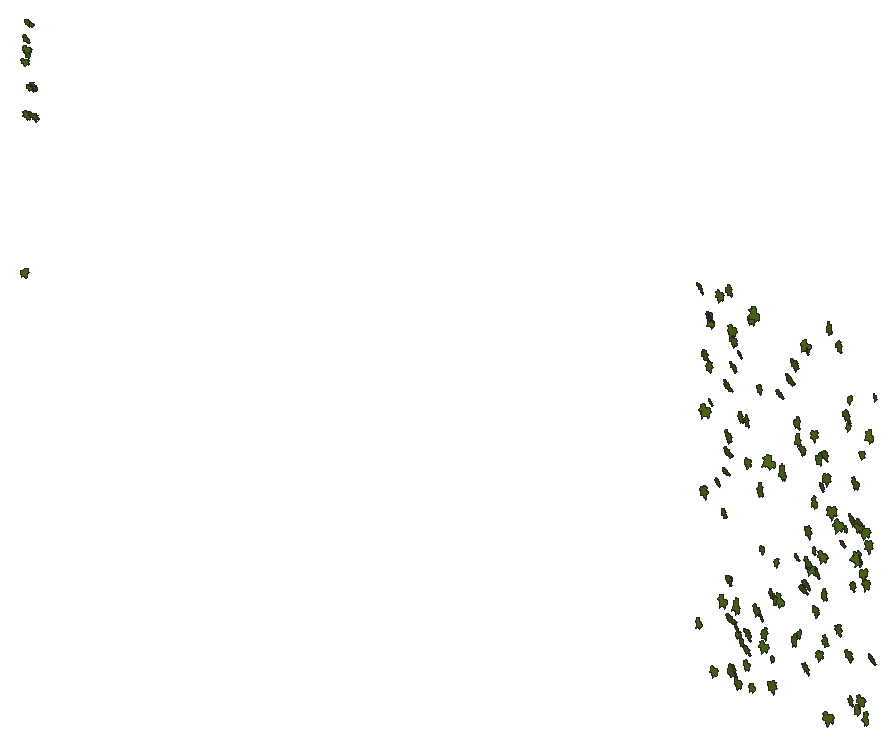
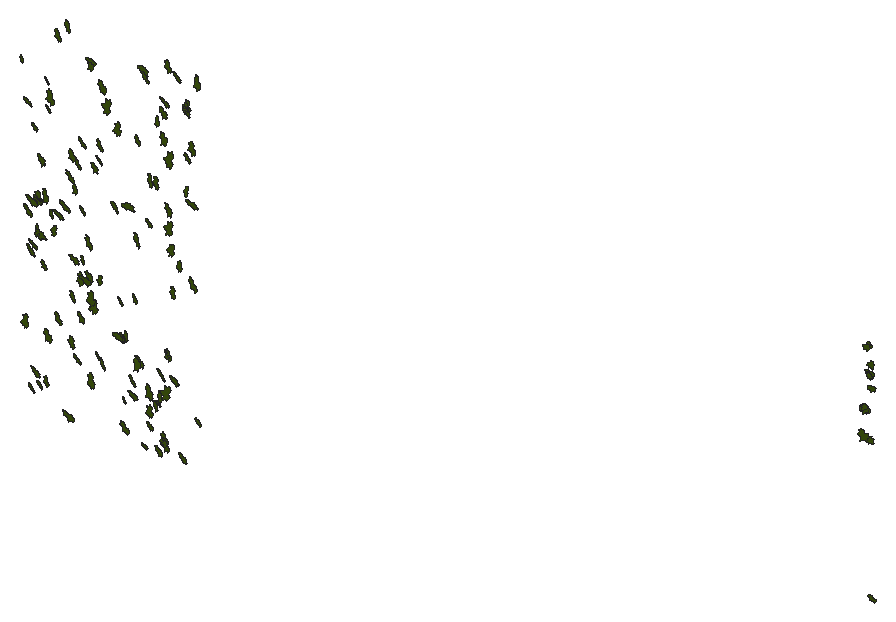
# SketchUp Ruby script. Lengths in inches.
U = 1.inch
M = Sketchup.active_model
def pt(a) = Geom::Point3d.new(a.map { |v| v * U })
def face(e, loops, mat)
  f = e.add_face(loops[0].map { |a| pt(a) })
  loops[1..].each { |l| e.add_face(l.map { |a| pt(a) }).erase! }
  f.material = f.back_material = mat if mat
  f
end
# faces: each face lists its corners as indices into pts; further lists are holes
def faces(e, pts, list, mat = nil) = list.each { |f| face(e, (f[0].is_a?(Array) ? f : [f]).map { |l| l.map { |i| pts[i] } }, mat) }
# xy, xz, yz: faces in a plane at the given z, y or x. An outline is a flat list of corners, or four numbers for a rectangle; further outlines are holes
def ring(l) = l.size == 4 ? [[l[0], l[1]], [l[2], l[1]], [l[2], l[3]], [l[0], l[3]]] : l.each_slice(2).to_a
def flat(e, list, mat, &to3) = list.each { |f| face(e, (f[0].is_a?(Array) ? f : [f]).map { |l| ring(l).map { |u, v| to3.(u, v) } }, mat) }
def xy(e, z, list, mat = nil) = flat(e, list, mat) { |x, y| [x, y, z] }
def xz(e, y, list, mat = nil) = flat(e, list, mat) { |x, z| [x, y, z] }
def yz(e, x, list, mat = nil) = flat(e, list, mat) { |y, z| [x, y, z] }
def lines(e, pts, list) = list.each { |a, b| e.add_line(pt(pts[a]), pt(pts[b])) }
# prism: a flat outline (further loops are holes) pulled along v
def prism(e, loops, v, mat = nil)
  f = face(e, loops, mat); d = Geom::Vector3d.new(v.map { |x| x * U })
  f.pushpull(f.normal.samedirection?(d) ? d.length : -d.length)
end
def box(e, o, s, mat = nil) = prism(e, [[o, [o[0] + s[0], o[1], o[2]], [o[0] + s[0], o[1] + s[1], o[2]], [o[0], o[1] + s[1], o[2]]]], [0, 0, s[2]], mat)
def at(x, y, z, deg = 0) = Geom::Transformation.translation(pt([x, y, z])) * Geom::Transformation.rotation(ORIGIN, Z_AXIS, deg.degrees)
def axes(o, x, y, z) = Geom::Transformation.new([*x, 0, *y, 0, *z, 0, *pt(o).to_a, 1])
def part(name) = M.definitions.add(name)
# library, detail: a bought-in or finely detailed component or shape, given as its bounding box
def library(name, o, s) = part(name).tap { |d| box(d.entities, o, s) }
def detail(e, o, s) = box(e.add_group.entities, o, s)
def put(e, d, t, mat = nil) = e.add_instance(d, t).tap { |i| i.material = mat if mat }
def group(e, t, mat = nil) = e.add_group.tap { |g| g.transformation = t; g.material = mat if mat }.entities
root = M.entities
M.materials.add("[Vegetation Blur 03]").color = [83, 114, 18]
c1 = part("ivy")
xy(c1.entities,0,[[0.782,0,0.786,0,0.787,0.005,0.789,0.009,0.821,0.072,0.875,0.147,1.001,0.272,1.073,0.331,1.137,0.363,1.178,0.379,1.223,0.384,1.272,0.383,1.311,0.374,1.36,0.355,1.399,0.334,1.491,0.285,1.541,0.244,1.583,0.199,1.617,0.15,1.64,0.128,1.662,0.115,1.717,0.105,1.745,0.093,1.784,0.054,1.819,0.057,1.854,0.064,1.882,0.075,1.896,0.074,1.91,0.071,1.937,0.063,1.964,0.053,1.99,0.038,2.016,0.015,2.034,0.002,2.04,0,2.038,0.003,2.036,0.007,2.033,0.038,2.036,0.068,2.045,0.1,2.055,0.116,2.064,0.123,2.077,0.129,2.088,0.129,2.106,0.132,2.118,0.13,2.179,0.132,2.207,0.133,2.225,0.133,2.242,0.138,2.22,0.162,2.207,0.186,2.206,0.213,2.212,0.236,2.228,0.262,2.247,0.274,2.298,0.283,2.355,0.294,2.37,0.296,2.376,0.295,2.377,0.3,2.377,0.303,2.385,0.329,2.411,0.37,2.426,0.392,2.449,0.407,2.511,0.426,2.561,0.444,2.619,0.466,2.589,0.469,2.561,0.476,2.501,0.5,2.449,0.516,2.424,0.523,2.401,0.535,2.377,0.556,2.372,0.568,2.36,0.575,2.268,0.586,2.225,0.592,2.207,0.599,2.194,0.61,2.143,0.65,2.13,0.664,2.122,0.682,2.123,0.7,2.13,0.719,2.148,0.75,2.17,0.781,2.195,0.807,2.221,0.828,2.284,0.874,2.291,0.88,2.288,0.887,2.276,0.9,2.267,0.916,2.265,0.933,2.273,0.967,2.292,1.002,2.313,1.03,2.334,1.054,2.348,1.067,2.358,1.074,2.363,1.076,2.362,1.081,2.35,1.094,2.347,1.11,2.35,1.143,2.359,1.18,2.385,1.254,2.415,1.324,2.448,1.393,2.45,1.4,2.446,1.398,2.44,1.394,2.427,1.383,2.402,1.36,2.376,1.339,2.345,1.324,2.305,1.309,2.282,1.303,2.273,1.306,2.245,1.294,2.212,1.287,2.187,1.291,2.163,1.301,2.142,1.316,2.134,1.327,2.124,1.325,2.09,1.292,2.053,1.259,2.014,1.234,1.973,1.215,1.954,1.21,1.931,1.208,1.909,1.212,1.893,1.22,1.879,1.233,1.872,1.248,1.867,1.281,1.864,1.319,1.821,1.258,1.773,1.197,1.726,1.141,1.698,1.121,1.679,1.116,1.666,1.117,1.647,1.122,1.632,1.129,1.62,1.141,1.617,1.154,1.617,1.219,1.621,1.254,1.623,1.268,1.623,1.281,1.618,1.314,1.606,1.346,1.603,1.375,1.607,1.403,1.603,1.467,1.599,1.499,1.605,1.525,1.614,1.552,1.629,1.577,1.635,1.589,1.629,1.587,1.618,1.582,1.596,1.566,1.581,1.556,1.568,1.552,1.557,1.55,1.545,1.553,1.531,1.562,1.522,1.572,1.504,1.591,1.486,1.611,1.474,1.631,1.457,1.666,1.455,1.684,1.457,1.698,1.452,1.715,1.444,1.728,1.424,1.754,1.419,1.772,1.423,1.786,1.434,1.819,1.444,1.848,1.446,1.855,1.44,1.861,1.43,1.867,1.386,1.904,1.349,1.948,1.326,1.973,1.31,1.995,1.288,2.048,1.284,2.153,1.287,2.254,1.284,2.255,1.282,2.253,1.278,2.247,1.274,2.237,1.266,2.216,1.226,2.125,1.208,2.076,1.184,2.033,1.155,1.984,1.135,1.942,1.111,1.899,1.083,1.861,1.053,1.85,1.059,1.83,1.061,1.809,1.056,1.79,1.049,1.767,1.04,1.749,1.018,1.733,0.994,1.726,0.942,1.734,0.95,1.6875,0.944,1.645,0.932,1.608,0.911,1.585,0.881,1.58,0.854,1.582,0.828,1.588,0.785,1.618,0.773,1.625,0.775,1.614,0.779,1.598,0.796,1.502,0.818,1.402,0.861,1.283,0.882,1.224,0.894,1.174,0.892,1.148,0.886,1.123,0.881,1.107,0.872,1.099,0.849,1.094,0.818,1.092,0.789,1.098,0.762,1.107,0.753,1.113,0.721,1.139,0.698,1.163,0.678,1.194,0.665,1.224,0.628,1.28,0.612,1.312,0.606,1.327,0.606,1.314,0.599,1.282,0.594,1.267,0.581,1.256,0.544,1.245,0.512,1.244,0.473,1.249,0.444,1.256,0.382,1.288,0.339,1.306,0.324,1.316,0.317,1.324,0.309,1.326,0.27,1.314,0.227,1.313,0.185,1.3125,0.152,1.317,0.122,1.328,0.092,1.345,0.073,1.353,0.079,1.338,0.092,1.308,0.117,1.249,0.13,1.215,0.139,1.164,0.147,1.148,0.157,1.136,0.163,1.122,0.174,1.086,0.177,1.067,0.182,1.054,0.186,1.043,0.191,1.038,0.211,1.028,0.237,1.005,0.25,0.974,0.253,0.96,0.25,0.944,0.242,0.914,0.243,0.906,0.249,0.902,0.26,0.894,0.289,0.88,0.307,0.873,0.322,0.862,0.364,0.799,0.403,0.738,0.431,0.709,0.439,0.691,0.441,0.678,0.4375,0.66,0.428,0.645,0.394,0.623,0.303,0.594,0.255,0.581,0.214,0.577,0.179,0.573,0.173,0.568,0.175,0.561,0.167,0.55,0.141,0.523,0.113,0.503,0.077,0.49,0.045,0.486,0.026,0.485,0.019,0.486,0.011,0.483,0,0.471,0.014,0.467,0.044,0.455,0.058,0.447,0.07,0.438,0.097,0.411,0.125,0.394,0.158,0.377,0.174,0.366,0.182,0.359,0.185,0.361,0.242,0.331,0.253,0.316,0.258,0.303,0.262,0.283,0.274,0.278,0.308,0.274,0.341,0.252,0.366,0.226,0.366,0.222,0.37,0.22,0.38,0.221,0.395,0.221,0.425,0.216,0.45,0.207,0.465,0.192,0.473,0.178,0.484,0.15,0.489,0.116,0.483,0.089,0.468,0.058,0.45,0.035,0.435,0.018,0.429,0.011,0.434,0.012,0.438,0.014,0.469,0.019,0.542,0.016,0.581,0.015,0.612,0.027,0.68,0.055,0.696,0.057,0.712,0.052,0.73,0.045,0.741,0.036,0.766,0.014]])
put(root,c1,axes([31.32,173.2,140.17],[0.36239,0.03439,0.0325],[0.04011,-0.01114,-0.29602],[0.01602,-0.75014,0.00588]),"[Vegetation Blur 03]")
put(root,c1,axes([31.76,173.2,143.07],[0.31224,-0.04153,-0.22289],[-0.2695,0.10455,-0.25454],[-0.04857,-0.84719,-0.02048]),"[Vegetation Blur 03]")
put(root,c1,axes([31.16,173.2,116.41],[0.30062,0.06409,0.25513],[0.31279,-0.14376,-0.23982],[-0.02918,-0.88082,0.05771]),"[Vegetation Blur 03]")
put(root,c1,axes([32.02,173.2,134.62],[0.2286,-0.00259,-0.27195],[-0.33307,0.02295,-0.18652],[-0.00991,-0.83122,-0.0043]),"[Vegetation Blur 03]")
put(root,c1,axes([32.45,173.2,141.72],[0.11758,-0.14394,-0.33997],[-0.41694,0.10295,-0.1029],[-0.06765,-0.88473,0.04334]),"[Vegetation Blur 03]")
put(root,c1,axes([31.58,173.2,141.8],[0.42779,-0.01722,0.00276],[0.0027,-0.07154,-0.34805],[-0.00862,-0.87743,0.02832]),"[Vegetation Blur 03]")
put(root,c1,axes([31.75,173.2,144.62],[0.24814,-0.07421,0.13501],[0.16554,-0.02052,-0.20443],[-0.03556,-0.61336,-0.0095]),"[Vegetation Blur 03]")
put(root,c1,axes([32.1,173.2,144.75],[0.32819,0.01887,-0.10221],[-0.12554,0.06541,-0.2666],[-0.0028,-0.71988,-0.0269]),"[Vegetation Blur 03]")
put(root,c1,axes([31.87,173.2,137.29],[0.29759,0.01634,0.29239],[0.3571,0.0663,-0.24267],[0.02985,-0.95609,-0.01183]),"[Vegetation Blur 03]")
put(root,c1,axes([32.18,173.2,137.7],[0.43208,-0.00485,-0.01137],[-0.01346,0.125,-0.34915],[-0.00429,-0.88078,-0.04949]),"[Vegetation Blur 03]")
put(root,c1,axes([32.07,173.2,134.58],[0.54527,-0.10858,0.11727],[0.14945,0.14116,-0.4423],[-0.03309,-1.15173,-0.06527]),"[Vegetation Blur 03]")
put(root,c1,axes([115.06,173.7,107.27],[0.44114,-0.2833,-0.10477],[-0.14493,-0.08165,-0.37173],[-0.12012,-0.94191,0.06374]),"[Vegetation Blur 03]")
put(root,c1,axes([114.86,173.7,144.42],[0.47356,-0.40672,0.26845],[0.33871,-0.06229,-0.41283],[-0.18036,-1.18486,-0.07045]),"[Vegetation Blur 03]")
put(root,c1,axes([115.53,173.7,131.28],[0.64635,-0.1795,-0.0483],[-0.07498,-0.25102,-0.52154],[-0.0741,-1.31182,0.10641]),"[Vegetation Blur 03]")
put(root,c1,axes([115.22,173.7,121.76],[0.52711,-0.21147,0.33505],[0.39283,-0.25745,-0.4372],[-0.15742,-1.35053,0.03088]),"[Vegetation Blur 03]")
put(root,c1,axes([115.43,173.7,136.7],[0.32628,-0.20206,0.40603],[0.49033,-0.18475,-0.27691],[-0.12932,-1.21026,-0.02552]),"[Vegetation Blur 03]")
put(root,c1,axes([116.1,173.7,141.6],[0.40522,-0.15446,0.13943],[0.15914,-0.15283,-0.3347],[-0.09744,-0.89194,0.0332]),"[Vegetation Blur 03]")
put(root,c1,axes([116.03,173.7,135.72],[0.34108,-0.07651,0.26436],[0.30846,-0.23678,-0.27587],[-0.10562,-0.93855,0.04805]),"[Vegetation Blur 03]")
put(root,c1,axes([116.6,173.7,141.49],[0.45619,-0.27219,-0.21417],[-0.27378,-0.03129,-0.38217],[-0.10679,-1.08253,0.0649]),"[Vegetation Blur 03]")
put(root,c1,axes([116.54,173.7,131.73],[0.12614,-0.2409,0.28031],[0.3435,-0.16191,-0.12485],[-0.11696,-0.73532,-0.06434]),"[Vegetation Blur 03]")
put(root,c1,axes([116.49,173.7,140.97],[0.11866,-0.26117,0.39663],[0.48542,-0.20436,-0.1179],[-0.12904,-1.00894,-0.07879]),"[Vegetation Blur 03]")
put(root,c1,axes([116.65,173.7,102.41],[0.52824,-0.2088,0.07813],[0.0803,-0.17577,-0.43551],[-0.11407,-1.09065,0.05523]),"[Vegetation Blur 03]")
put(root,c1,axes([117.2,173.7,123.2],[0.23432,-0.21265,0.28086],[0.3439,-0.11223,-0.20448],[-0.10411,-0.84934,-0.0433]),"[Vegetation Blur 03]")
put(root,c1,axes([117.39,173.7,144.48],[0.53111,-0.22481,0.11811],[0.12292,-0.23121,-0.43739],[-0.1333,-1.10892,0.06725]),"[Vegetation Blur 03]")
put(root,c1,axes([117.9,173.7,110.91],[0.58633,-0.27865,-0.1062],[-0.1477,-0.14213,-0.48453],[-0.11598,-1.22771,0.08019]),"[Vegetation Blur 03]")
put(root,c1,axes([117.98,173.7,119.81],[0.1731,-0.14266,0.38005],[0.45428,-0.21748,-0.15066],[-0.12362,-0.99891,-0.02148]),"[Vegetation Blur 03]")
put(root,c1,axes([118.19,173.7,124.49],[0.13916,-0.21976,0.37305],[0.46529,-0.06512,-0.12164],[-0.06205,-0.98109,-0.07549]),"[Vegetation Blur 03]")
put(root,c1,axes([118.49,173.7,126.62],[0.10022,-0.2222,0.4688],[0.57871,-0.13035,-0.09212],[-0.08191,-1.19279,-0.07727]),"[Vegetation Blur 03]")
put(root,c1,axes([118.39,173.7,129.41],[0.62179,-0.3866,0.07255],[0.08725,-0.03824,-0.53009],[-0.18864,-1.29198,-0.00602]),"[Vegetation Blur 03]")
put(root,c1,axes([118.45,173.7,112.9],[0.37075,-0.20222,0.27738],[0.33431,-0.13128,-0.31269],[-0.11578,-1.02663,-0.01465]),"[Vegetation Blur 03]")
put(root,c1,axes([118.4375,173.7,144.87],[0.27432,-0.11887,0.39101],[0.46845,-0.2067,-0.22879],[-0.11587,-1.1171,0.00072]),"[Vegetation Blur 03]")
put(root,c1,axes([118.4,173.7,134.14],[0.18149,-0.29755,0.51892],[0.63719,-0.20751,-0.16715],[-0.13848,-1.34475,-0.08903]),"[Vegetation Blur 03]")
put(root,c1,axes([118.8,173.7,112.98],[0.30081,-0.15518,0.1985],[0.21889,-0.23826,-0.25024],[-0.13012,-0.75955,0.03794]),"[Vegetation Blur 03]")
put(root,c1,axes([118.8125,173.7,108.14],[0.09309,-0.2572,0.47512],[0.59358,-0.05541,-0.08218],[-0.0469,-1.21192,-0.09707]),"[Vegetation Blur 03]")
put(root,c1,axes([118.6875,173.7,102.4],[0.19741,-0.09695,0.50499],[0.60705,-0.24693,-0.16553],[-0.12869,-1.3135,-0.00615]),"[Vegetation Blur 03]")
put(root,c1,axes([118.93,173.7,141.25],[0.5878,-0.24093,0.03931],[0.02588,-0.23212,-0.48155],[-0.12393,-1.19122,0.08588]),"[Vegetation Blur 03]")
put(root,c1,axes([118.9375,173.7,137.15],[0.5598,-0.34639,0.09978],[0.13771,0.07562,-0.47332],[-0.15594,-1.17668,-0.05979]),"[Vegetation Blur 03]")
put(root,c1,axes([119,173.7,140.08],[0.56579,-0.26175,0.06944],[0.08066,-0.05979,-0.47321],[-0.13005,-1.17586,0.0086]),"[Vegetation Blur 03]")
put(root,c1,axes([119.02,173.7,103.04],[0.3696,-0.27711,0.38105],[0.45779,-0.2062,-0.31935],[-0.16294,-1.2079,-0.0329]),"[Vegetation Blur 03]")
put(root,c1,axes([119.96,173.7,111.21],[0.5074,-0.4678,-0.2898],[-0.37384,0.02954,-0.44347],[-0.19497,-1.27408,0.09613]),"[Vegetation Blur 03]")
put(root,c1,axes([119.83,173.7,107.24],[0.27201,-0.08351,0.1346],[0.14493,-0.22002,-0.21655],[-0.08857,-0.61651,0.05905]),"[Vegetation Blur 03]")
put(root,c1,axes([119.73,173.7,107.69],[0.16819,-0.22664,0.32974],[0.39401,-0.21788,-0.15742],[-0.14187,-0.87383,-0.04627]),"[Vegetation Blur 03]")
put(root,c1,axes([119.64,173.7,102.19],[0.53858,-0.252,0.05397],[0.05479,-0.1161,-0.44944],[-0.12794,-1.11057,0.03474]),"[Vegetation Blur 03]")
put(root,c1,axes([119.98,173.7,138.58],[0.31604,-0.28517,0.16056],[0.20748,-0.01555,-0.27638],[-0.12189,-0.7659,-0.05417]),"[Vegetation Blur 03]")
put(root,c1,axes([120.3,173.7,107.26],[0.4884,-0.38994,-0.09349],[-0.11293,0.05241,-0.42733],[-0.19047,-1.03097,0.01363]),"[Vegetation Blur 03]")
put(root,c1,axes([120.05,173.7,131.25],[0.21062,-0.15839,0.41958],[0.49728,-0.27124,-0.18238],[-0.15148,-1.11064,-0.0153]),"[Vegetation Blur 03]")
put(root,c1,axes([120.87,173.7,104.6],[0.49081,-0.25055,0.00673],[-0.00728,-0.13032,-0.40947],[-0.12182,-1.0017,0.05159]),"[Vegetation Blur 03]")
put(root,c1,axes([120.72,173.7,105.65],[0.28606,-0.20547,0.36321],[0.44363,-0.1257,-0.24391],[-0.10592,-1.08138,-0.04066]),"[Vegetation Blur 03]")
put(root,c1,axes([120.91,173.7,127.01],[0.44605,-0.17185,0.11357],[0.12178,-0.19918,-0.36599],[-0.10728,-0.94065,0.05675]),"[Vegetation Blur 03]")
put(root,c1,axes([120.78,173.7,131.1875],[0.25712,-0.18798,0.42224],[0.4923,-0.32764,-0.22263],[-0.18343,-1.14283,-0.00563]),"[Vegetation Blur 03]")
put(root,c1,axes([120.73,173.7,107.98],[0.55958,-0.3731,0.26041],[0.3198,-0.09162,-0.47837],[-0.18004,-1.32239,-0.04033]),"[Vegetation Blur 03]")
put(root,c1,axes([121.6875,173.7,102.27],[0.36884,-0.18268,-0.08765],[-0.12074,-0.10682,-0.30338],[-0.06956,-0.78327,0.06182]),"[Vegetation Blur 03]")
put(root,c1,axes([121.17,173.7,142.66],[0.3032,0.00804,0.42723],[0.50376,-0.343,-0.23711],[-0.14236,-1.19666,0.07083]),"[Vegetation Blur 03]")
put(root,c1,axes([122.01,173.7,144.4],[0.54958,-0.28156,-0.28314],[-0.3622,-0.10008,-0.45262],[-0.08884,-1.33367,0.09374]),"[Vegetation Blur 03]")
put(root,c1,axes([121.97,173.7,111.18],[0.5531,-0.30937,0.07702],[0.082,-0.11827,-0.46698],[-0.15743,-1.14854,0.02734]),"[Vegetation Blur 03]")
put(root,c1,axes([122.3,173.7,135.49],[0.34266,-0.16677,0.2483],[0.29126,-0.18349,-0.28712],[-0.11956,-0.92493,0.01219]),"[Vegetation Blur 03]")
put(root,c1,axes([122.31,173.7,110.93],[0.62192,-0.51222,0.08279],[0.13225,0.12501,-0.54004],[-0.23401,-1.29066,-0.08517]),"[Vegetation Blur 03]")
put(root,c1,axes([122.38,173.7,123.84],[0.18528,-0.05644,0.53215],[0.61865,-0.42892,-0.15063],[-0.2078,-1.32731,0.02605]),"[Vegetation Blur 03]")
put(root,c1,axes([122.76,173.7,117.9],[0.3651,-0.20886,0.13721],[0.15459,-0.14475,-0.30864],[-0.12111,-0.81437,0.01967]),"[Vegetation Blur 03]")
put(root,c1,axes([122.87,173.7,107.41],[0.56213,-0.17838,-0.00831],[-0.02255,-0.16495,-0.45927],[-0.08432,-1.14512,0.06745]),"[Vegetation Blur 03]")
put(root,c1,axes([122.9,173.7,108.37],[0.33688,-0.08622,0.33874],[0.38873,-0.33347,-0.27086],[-0.15137,-1.04826,0.0583]),"[Vegetation Blur 03]")
put(root,c1,axes([123.91,173.7,128.56],[0.49181,-0.15671,-0.3315],[-0.41314,-0.21702,-0.39213],[0.00973,-1.29451,0.10587]),"[Vegetation Blur 03]")
put(root,c1,axes([123.92,173.7,112.97],[0.15407,-0.1087,0.33806],[0.39127,-0.27976,-0.13293],[-0.14585,-0.86534,0.00051]),"[Vegetation Blur 03]")
put(root,c1,axes([124.18,173.7,106.15],[0.27567,-0.18278,0.07916],[0.08,-0.13493,-0.23455],[-0.1044,-0.58604,0.02931]),"[Vegetation Blur 03]")
put(root,c1,axes([123.63,173.7,102.98],[0.51611,-0.14167,0.29822],[0.35265,-0.22138,-0.42305],[-0.1179,-1.28232,0.04009]),"[Vegetation Blur 03]")
put(root,c1,axes([124.38,173.7,113.2],[0.43914,-0.29657,0.03896],[0.03337,-0.10478,-0.37595],[-0.14811,-0.90294,0.03083]),"[Vegetation Blur 03]")
put(root,c1,axes([124.51,173.7,116.86],[0.29156,-0.09126,0.22735],[0.25627,-0.25873,-0.23525],[-0.11785,-0.78843,0.05088]),"[Vegetation Blur 03]")
put(root,c1,axes([125.12,173.7,113.54],[0.50163,-0.24569,-0.26541],[-0.34021,-0.12729,-0.40976],[-0.06534,-1.2236,0.09592]),"[Vegetation Blur 03]")
put(root,c1,axes([124.75,173.7,135.72],[0.30187,-0.29092,0.34167],[0.43037,-0.04293,-0.25902],[-0.10016,-1.06123,-0.08319]),"[Vegetation Blur 03]")
put(root,c1,axes([125.66,173.7,128.05],[0.48032,-0.40321,-0.3461],[-0.42858,0.11763,-0.41773],[-0.18586,-1.31325,0.06885]),"[Vegetation Blur 03]")
put(root,c1,axes([126.23,173.7,137.39],[0.07798,-0.22712,0.49701],[0.61066,-0.17712,-0.07655],[-0.10063,-1.25091,-0.0794]),"[Vegetation Blur 03]")
put(root,c1,axes([126.5,173.7,140.07],[0.58958,-0.29849,0.19052],[0.22934,-0.09222,-0.49546],[-0.15145,-1.30163,-0.00859]),"[Vegetation Blur 03]")
put(root,c1,axes([126.63,173.7,108.75],[0.26152,-0.04302,0.44662],[0.5117,-0.42542,-0.20602],[-0.19512,-1.17335,0.05832]),"[Vegetation Blur 03]")
put(root,c1,axes([127.14,173.7,118.17],[0.15681,-0.19135,0.27864],[0.34217,-0.11382,-0.14055],[-0.09017,-0.7647,-0.0488]),"[Vegetation Blur 03]")
put(root,c1,axes([126.93,173.7,133.11],[0.28904,-0.06987,0.39444],[0.46239,-0.30604,-0.23421],[-0.14468,-1.11768,0.03947]),"[Vegetation Blur 03]")
put(root,c1,axes([127.56,173.7,132.16],[0.42016,-0.3703,-0.17602],[-0.23818,-0.04638,-0.36333],[-0.14889,-0.97076,0.0845]),"[Vegetation Blur 03]")
put(root,c1,axes([127.36,173.7,109.79],[0.24227,-0.06001,0.24324],[0.27574,-0.26297,-0.19314],[-0.11679,-0.74533,0.04856]),"[Vegetation Blur 03]")
put(root,c1,axes([127.63,173.7,130.96],[0.51145,-0.25079,0.06105],[0.06998,-0.0596,-0.42899],[-0.12471,-1.06199,0.00966]),"[Vegetation Blur 03]")
put(root,c1,axes([127.61,173.7,114.92],[0.32867,-0.28906,0.36046],[0.45664,0.0115,-0.27589],[-0.07923,-1.13284,-0.09478]),"[Vegetation Blur 03]")
put(root,c1,axes([128.24,173.7,142.85],[0.51677,-0.16,-0.11108],[-0.14975,-0.2188,-0.41446],[-0.04632,-1.0777,0.10064]),"[Vegetation Blur 03]")
put(root,c1,axes([128.12,173.7,142.01],[0.40968,-0.27629,0.16507],[0.21084,0.00024,-0.34848],[-0.12034,-0.94019,-0.0486]),"[Vegetation Blur 03]")
put(root,c1,axes([127.94,173.7,115.6875],[0.38346,-0.30784,0.36497],[0.45646,-0.05536,-0.32679],[-0.11835,-1.21097,-0.07784]),"[Vegetation Blur 03]")
put(root,c1,axes([128.41,173.7,118.82],[0.56324,-0.31646,-0.09717],[-0.11977,0.02711,-0.47626],[-0.15324,-1.18433,0.01506]),"[Vegetation Blur 03]")
put(root,c1,axes([127.96,173.7,106.5],[0.44878,-0.3413,0.36007],[0.4395,-0.14984,-0.38721],[-0.17027,-1.28634,-0.05043]),"[Vegetation Blur 03]")
put(root,c1,axes([128.26,173.7,121.87],[0.47957,-0.26061,0.31785],[0.37221,-0.23733,-0.40467],[-0.1708,-1.24893,0.01057]),"[Vegetation Blur 03]")
put(root,c1,axes([128.76,173.7,118.26],[0.59751,-0.1415,-0.08723],[-0.11552,-0.16395,-0.48523],[-0.05298,-1.23827,0.07421]),"[Vegetation Blur 03]")
put(root,c1,axes([129.55,173.7,125.92],[0.4464,-0.35085,-0.18371],[-0.23796,-0.0009,-0.38487],[-0.15203,-1.02878,0.06299]),"[Vegetation Blur 03]")
put(root,c1,axes([129.26,173.7,119.75],[0.21308,-0.12887,0.25392],[0.29486,-0.2048,-0.18116],[-0.11737,-0.74847,0.00585]),"[Vegetation Blur 03]")
put(root,c1,axes([129.1,173.7,132.9],[0.46976,-0.15316,0.21327],[0.23871,-0.28032,-0.3819],[-0.12977,-1.07007,0.06952]),"[Vegetation Blur 03]")
put(root,c1,axes([129.29,173.7,113.51],[0.49387,-0.24848,0.14861],[0.17062,-0.13992,-0.41447],[-0.13648,-1.07408,0.01961]),"[Vegetation Blur 03]")
put(root,c1,axes([129.4,173.7,117.45],[0.34584,-0.27967,0.31588],[0.38688,-0.124,-0.2994],[-0.13639,-1.06088,-0.04828]),"[Vegetation Blur 03]")
put(root,c1,axes([129.66,173.7,130.13],[0.31073,-0.06738,0.37222],[0.4328,-0.32267,-0.24985],[-0.14749,-1.08882,0.05101]),"[Vegetation Blur 03]")
put(root,c1,axes([129.79,173.7,108.68],[0.45593,-0.14871,0.15697],[0.17169,-0.25336,-0.36992],[-0.11285,-0.98625,0.07136]),"[Vegetation Blur 03]")
put(root,c1,axes([130.1,173.7,127.4375],[0.37901,-0.24998,0.16924],[0.20826,-0.05609,-0.32368],[-0.11995,-0.88726,-0.02722]),"[Vegetation Blur 03]")
put(root,c1,axes([130.1,173.7,119.98],[0.58607,-0.17658,0.01299],[0.00501,-0.15402,-0.47969],[-0.08713,-1.19658,0.05983]),"[Vegetation Blur 03]")
put(root,c1,axes([130.4,173.7,114.98],[0.16191,-0.03187,0.41572],[0.48687,-0.31523,-0.1301],[-0.15054,-1.05373,0.02635]),"[Vegetation Blur 03]")
put(root,c1,axes([130.36,173.7,130.95],[0.39018,-0.19806,0.28181],[0.33951,-0.13277,-0.32778],[-0.115,-1.06391,-0.01155]),"[Vegetation Blur 03]")
put(root,c1,axes([130.5,173.7,109.8125],[0.12637,-0.06641,0.44261],[0.52763,-0.25805,-0.10643],[-0.12947,-1.11645,-0.00173]),"[Vegetation Blur 03]")
put(root,c1,axes([130.51,173.7,128.55],[0.51632,-0.17161,0.26126],[0.29868,-0.283,-0.42241],[-0.14219,-1.21766,0.06135]),"[Vegetation Blur 03]")
put(root,c1,axes([130.65,173.7,102.21],[0.65317,-0.15035,0.08957],[0.09783,-0.2124,-0.5313],[-0.08838,-1.34629,0.07382]),"[Vegetation Blur 03]")
put(root,c1,axes([131.04,173.7,144.75],[0.0835,-0.00667,0.46395],[0.54474,-0.33722,-0.06606],[-0.16259,-1.13325,0.01693]),"[Vegetation Blur 03]")
put(root,c1,axes([131.07,173.7,125.15],[0.58365,-0.1286,0.23072],[0.26562,-0.28309,-0.47237],[-0.11521,-1.30414,0.07979]),"[Vegetation Blur 03]")
put(root,c1,axes([132.16,173.7,124.24],[0.61381,-0.2023,0.00115],[-0.01893,-0.26118,-0.49641],[-0.09648,-1.23581,0.10472]),"[Vegetation Blur 03]")
put(root,c1,axes([132.04,173.7,112.1],[0.40591,-0.18014,0.3374],[0.39655,-0.24525,-0.33836],[-0.14603,-1.16675,0.01903]),"[Vegetation Blur 03]")
put(root,c1,axes([132.16,173.7,143.55],[0.32606,-0.15993,0.37004],[0.43652,-0.25327,-0.27342],[-0.14515,-1.12098,0.00898]),"[Vegetation Blur 03]")
put(root,c1,axes([132.91,173.7,121.57],[0.07402,-0.1812,0.31745],[0.39109,-0.12634,-0.07209],[-0.07805,-0.80492,-0.06015]),"[Vegetation Blur 03]")
put(root,c1,axes([133.18,173.7,123.51],[0.18332,-0.13201,0.23981],[0.28131,-0.17522,-0.15841],[-0.10639,-0.6908,-0.00565]),"[Vegetation Blur 03]")
put(root,c1,axes([132.99,173.7,136.22],[0.41734,-0.25524,0.42347],[0.50918,-0.21404,-0.35453],[-0.15923,-1.35344,-0.02379]),"[Vegetation Blur 03]")
put(root,c1,axes([133.58,173.7,135.36],[0.35292,-0.17211,0.08002],[0.07901,-0.17569,-0.29156],[-0.10181,-0.73298,0.0511]),"[Vegetation Blur 03]")
put(root,c1,axes([133.28,173.7,110.03],[0.57796,-0.29472,0.19025],[0.2281,-0.10009,-0.48593],[-0.15109,-1.27852,-0.00582]),"[Vegetation Blur 03]")
put(root,c1,axes([133.71,173.7,138.2],[0.24496,-0.07431,0.21292],[0.23492,-0.26987,-0.19483],[-0.11909,-0.6852,0.05364]),"[Vegetation Blur 03]")
put(root,c1,axes([133.69,173.7,104.52],[0.23742,-0.1267,0.33587],[0.39552,-0.23419,-0.20013],[-0.12927,-0.94922,0.00454]),"[Vegetation Blur 03]")
put(root,c1,axes([133.93,173.7,117.59],[0.33061,-0.13828,0.23143],[0.27228,-0.16795,-0.27487],[-0.10387,-0.88042,0.01609]),"[Vegetation Blur 03]")
put(root,c1,axes([133.72,173.7,125.38],[0.56286,-0.41503,0.17137],[0.21267,-0.05627,-0.48669],[-0.19885,-1.23496,-0.03542]),"[Vegetation Blur 03]")
put(root,c1,axes([134.26,173.7,129.7],[0.59158,-0.31026,-0.0564],[-0.07139,-0.00087,-0.49803],[-0.1497,-1.22563,0.01463]),"[Vegetation Blur 03]")
put(root,c1,axes([135.26,173.7,121.6875],[0.30037,-0.23448,-0.48095],[-0.59958,-0.05449,-0.24524],[-0.02777,-1.36002,0.09275]),"[Vegetation Blur 03]")
put(root,c1,axes([134.8125,173.7,104.57],[0.42261,-0.28747,-0.1193],[-0.16204,-0.06467,-0.35783],[-0.12093,-0.91792,0.06257]),"[Vegetation Blur 03]")
put(root,c1,axes([134.7,173.7,124.92],[0.52102,-0.20474,0.04178],[0.03433,-0.18504,-0.42777],[-0.1065,-1.06132,0.06652]),"[Vegetation Blur 03]")
put(root,c1,axes([134.49,173.7,124.59],[0.31137,-0.19726,0.4006],[0.48849,-0.13513,-0.26337],[-0.10722,-1.1885,-0.03655]),"[Vegetation Blur 03]")
put(root,c1,axes([134.92,173.7,121.04],[0.31064,-0.27454,0.24989],[0.28954,-0.20759,-0.27561],[-0.1665,-0.87322,-0.01304]),"[Vegetation Blur 03]")
put(root,c1,axes([134.9,173.7,105.62],[0.59208,-0.24793,0.06374],[0.06017,-0.19072,-0.48897],[-0.13036,-1.21404,0.0638]),"[Vegetation Blur 03]")
put(root,c1,axes([135.13,173.7,132.73],[0.36627,-0.13941,0.12421],[0.13945,-0.15724,-0.30166],[-0.09113,-0.8009,0.0376]),"[Vegetation Blur 03]")
put(root,c1,axes([135.14,173.7,119.55],[0.46252,-0.08041,0.20679],[0.23593,-0.28736,-0.36906],[-0.10033,-1.0465,0.08545]),"[Vegetation Blur 03]")
put(root,c1,axes([136.17,173.7,104.15],[0.33567,-0.36714,-0.32626],[-0.40941,0.10373,-0.29893],[-0.15499,-1.06915,0.08303]),"[Vegetation Blur 03]")
put(root,c1,axes([135.26,173.7,124.58],[0.64177,-0.16774,0.0763],[0.07979,-0.21804,-0.52237],[-0.09498,-1.31665,0.07678]),"[Vegetation Blur 03]")
put(root,c1,axes([135.58,173.7,118.9],[0.57824,-0.2854,0.09144],[0.09076,-0.20234,-0.48162],[-0.15346,-1.19504,0.05971]),"[Vegetation Blur 03]")
put(root,c1,axes([136.47,173.7,135.75],[0.44457,-0.30415,-0.24459],[-0.31847,-0.07486,-0.37092],[-0.10118,-1.10076,0.09281]),"[Vegetation Blur 03]")
put(root,c1,axes([135.76,173.7,122.98],[0.53293,-0.19106,0.2627],[0.2994,-0.28671,-0.43737],[-0.15029,-1.24869,0.06023]),"[Vegetation Blur 03]")
put(root,c1,axes([136.25,173.7,110.26],[0.31828,-0.32105,0.3684],[0.45752,-0.11523,-0.27908],[-0.137,-1.13071,-0.07616]),"[Vegetation Blur 03]")
put(root,c1,axes([136.87,173.7,139.74],[0.30667,-0.21087,0.08542],[0.09735,-0.07998,-0.26385],[-0.10945,-0.662,0.00467]),"[Vegetation Blur 03]")
